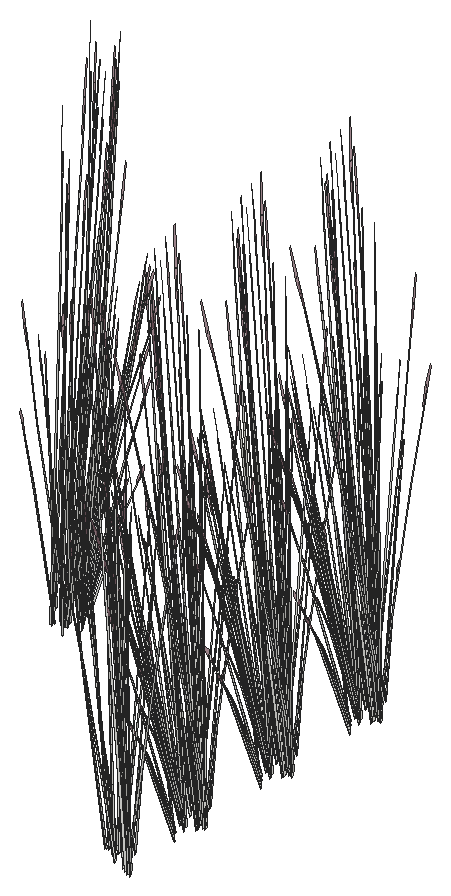
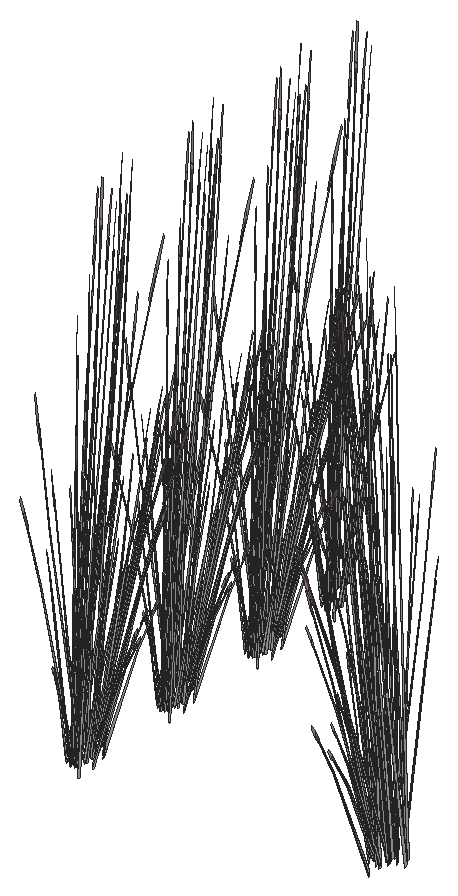
# SketchUp Ruby script. Lengths in inches.
U = 1.inch
M = Sketchup.active_model
def pt(a) = Geom::Point3d.new(a.map { |v| v * U })
def face(e, loops, mat)
  f = e.add_face(loops[0].map { |a| pt(a) })
  loops[1..].each { |l| e.add_face(l.map { |a| pt(a) }).erase! }
  f.material = f.back_material = mat if mat
  f
end
# faces: each face lists its corners as indices into pts; further lists are holes
def faces(e, pts, list, mat = nil) = list.each { |f| face(e, (f[0].is_a?(Array) ? f : [f]).map { |l| l.map { |i| pts[i] } }, mat) }
# xy, xz, yz: faces in a plane at the given z, y or x. An outline is a flat list of corners, or four numbers for a rectangle; further outlines are holes
def ring(l) = l.size == 4 ? [[l[0], l[1]], [l[2], l[1]], [l[2], l[3]], [l[0], l[3]]] : l.each_slice(2).to_a
def flat(e, list, mat, &to3) = list.each { |f| face(e, (f[0].is_a?(Array) ? f : [f]).map { |l| ring(l).map { |u, v| to3.(u, v) } }, mat) }
def xy(e, z, list, mat = nil) = flat(e, list, mat) { |x, y| [x, y, z] }
def xz(e, y, list, mat = nil) = flat(e, list, mat) { |x, z| [x, y, z] }
def yz(e, x, list, mat = nil) = flat(e, list, mat) { |y, z| [x, y, z] }
def lines(e, pts, list) = list.each { |a, b| e.add_line(pt(pts[a]), pt(pts[b])) }
# prism: a flat outline (further loops are holes) pulled along v
def prism(e, loops, v, mat = nil)
  f = face(e, loops, mat); d = Geom::Vector3d.new(v.map { |x| x * U })
  f.pushpull(f.normal.samedirection?(d) ? d.length : -d.length)
end
def box(e, o, s, mat = nil) = prism(e, [[o, [o[0] + s[0], o[1], o[2]], [o[0] + s[0], o[1] + s[1], o[2]], [o[0], o[1] + s[1], o[2]]]], [0, 0, s[2]], mat)
def at(x, y, z, deg = 0) = Geom::Transformation.translation(pt([x, y, z])) * Geom::Transformation.rotation(ORIGIN, Z_AXIS, deg.degrees)
def axes(o, x, y, z) = Geom::Transformation.new([*x, 0, *y, 0, *z, 0, *pt(o).to_a, 1])
def part(name) = M.definitions.add(name)
# library, detail: a bought-in or finely detailed component or shape, given as its bounding box
def library(name, o, s) = part(name).tap { |d| box(d.entities, o, s) }
def detail(e, o, s) = box(e.add_group.entities, o, s)
def put(e, d, t, mat = nil) = e.add_instance(d, t).tap { |i| i.material = mat if mat }
def group(e, t, mat = nil) = e.add_group.tap { |g| g.transformation = t; g.material = mat if mat }.entities
root = M.entities
M.materials.add("LightPink_Translucent").color = [144, 107, 117]
M.materials["LightPink_Translucent"].alpha = 0.75
c1 = part("blade")
p = [[2.15,0.21,22],[0,0.17,0],[0.09,0.45,0],[2.18,0.31,22],[2.29,0.31,22],[0.38,0.45,0],
  [2.48,0.24,33],[2.49,0.24,33],[2.48,0.22,33]]
faces(c1.entities,p,[[0,1,2,3],[4,5,2,3],[6,3,4,7],[8,0,3,6]])
c2 = part("seeds")
p = [[0.3,-0.1,1.38],[-0.01,-0.03,1.59],[-0.01,-0.03,0.03],[0.14,-0.07,-0.07],[0.29,-0.03,3],[0.15,0.01,3.11]]
faces(c2.entities,p,[[0,1,2,3],[1,0,4,5]],"LightPink_Translucent")
c3 = part("blade with seeds")
put(c3.entities,c1,at(0,0,0))
put(c3.entities,c2,axes([2.4,0.25,30.99],[1.5799,-0.05474,1.17369],[-0.12525,1.92788,0.29478],[-0.07173,-0.02425,1.56792]))
put(root,c3,axes([400.33,754.45,4.53],[-0.29332,-0.1301,-0.35414],[0.08555,-0.37955,0.4572],[-0.11809,0.0348,0.87481]))
put(root,c3,axes([401.96,755.35,2.67],[-0.35635,0.30962,-0.29095],[-0.23697,-0.43749,-0.50002],[-0.08792,-0.04443,1.59708]))
put(root,c3,axes([401.93,755.49,2.62],[-0.06809,0.4162,0.1448],[-0.33266,-0.07225,-0.41347],[-0.06054,-0.04274,1.26744]))
put(root,c3,axes([401.22,754.38,3.34],[0.10032,-0.06746,1.77064],[0.0346,0.47103,0.13857],[-0.2173,0.0625,0.63284]))
put(root,c3,axes([402.36,755.49,2.46],[-0.34464,-0.37536,-0.25192],[0.29,-0.42149,0.5513],[-0.0928,0.04391,1.68216]))
put(root,c3,axes([401.45,756.21,2.48],[0.33032,0.23318,0.49651],[-0.19744,0.41812,0],[-0.07523,-0.05311,1.57504]))
put(root,c3,axes([400.53,754.64,4.68],[-0.09562,0.42421,-0.51099],[-0.32782,-0.1454,-0.3958],[-0.13199,0.0389,0.97773]))
put(root,c3,axes([401.26,756.46,2.375],[-0.22066,0.46731,0],[-0.36918,-0.26061,-0.51607],[-0.08408,-0.05936,1.63711]))
put(root,c3,axes([402.1875,755.41,2.21],[-0.38326,0.02879,-0.44739],[-0.03466,-0.47788,0.21531],[-0.06861,0.04843,1.43643]))
put(root,c3,axes([400.52,754.86,3.875],[0.12246,-0.09864,1.71376],[0.1031,0.45582,0.13857],[-0.19225,0.10302,0.73262]))
put(root,c3,axes([400.14,755.64,2.59],[0.12266,0.03828,1.43002],[0.07906,0.39104,-0.30754],[-0.16661,0.0732,0.61141]))
put(root,c3,axes([399.88,756.46,2.77],[0.14709,-0.21136,1.1486],[0.05804,0.3346,0.84392],[-0.1063,0.05991,0.25299]))
put(root,c3,axes([400.43,755.54,4.53],[-0.30722,0.06665,-0.35414],[-0.08112,-0.381,0.4572],[-0.08804,0.10234,0.87481]))
put(root,c3,axes([402.2,755.6875,2.06],[-0.23773,0.35053,-0.62353],[-0.29532,-0.31785,-0.16365],[-0.09526,0.08744,1.37633]))
put(root,c3,axes([400.97,755.17,3.875],[0.08815,-0.14329,1.71376],[0.22258,0.38678,0.13857],[-0.15267,0.17614,0.73262]))
put(root,c3,axes([400.6875,755.59,4.68],[0.09067,0.42583,-0.51099],[-0.34336,0.07449,-0.3958],[-0.0984,0.11438,0.97773]))
put(root,c3,axes([400.27,756.67,1.49],[0.04734,0.04659,1.76342],[0.08027,0.4317,-0.26939],[-0.10492,0.09206,0.30037]))
put(root,c3,axes([400.9,755.52,3.875],[0.06572,-0.16029,1.71376],[0.27569,0.33172,0.13857],[-0.12437,0.20675,0.73262]))
put(root,c3,axes([400.98,756.42,4.53],[-0.23881,0.24554,-0.35414],[-0.22606,-0.28036,0.4572],[-0.0344,0.14245,0.87481]))
put(root,c3,axes([401.13,757.38,2.77],[-0.00913,-0.2773,1.1486],[0.22824,0.19778,0.84392],[-0.04489,0.13217,0.25299]))
put(root,c3,axes([401.27,763.66,3.875],[0.08068,0.14973,1.71376],[-0.3728,0.12606,0.13857],[-0.08426,-0.23506,0.73262]))
put(root,c3,axes([401.17,763.26,2.59],[-0.02137,0.15256,1.43002],[-0.31245,0.12771,-0.30754],[-0.07303,-0.19719,0.61141]))
put(root,c3,axes([401.13,756.16,5.34],[-0.00918,0.43138,-0.7886],[-0.38672,-0.02897,0.09517],[-0.04081,0.18275,1.11556]))
put(root,c3,axes([400.86,757.13,2.59],[0.11138,-0.07357,1.43002],[0.27499,0.22183,-0.30754],[-0.08185,0.19194,0.61141]))
put(root,c3,axes([401.0625,763.01,2.77],[0.18411,0.16231,1.1486],[-0.26813,0.09757,0.84392],[-0.05737,-0.12474,0.25299]))
put(root,c3,axes([401.51,763.875,4.98],[-0.30095,-0.22541,-0.71045],[0.21388,-0.395,0.08574],[-0.10904,-0.13459,1.00501]))
put(root,c3,axes([401.4,763.58,4.53],[-0.05451,-0.37564,-0.35414],[0.31161,-0.09919,0.4572],[-0.0837,-0.10765,0.87481]))
put(root,c3,axes([401.01,756.77,3.36],[0.00775,-0.24075,1.54345],[0.34877,0.12716,0.21329],[-0.03022,0.25658,0.72882]))
put(root,c3,axes([400.92,763.5,1.49],[-0.03419,0.06144,1.76342],[-0.3455,0.13246,-0.26939],[-0.08346,-0.12049,0.30037]))
put(root,c3,axes([400.73,764.12,3.875],[0.1311,0.08035,1.71376],[-0.27131,0.33708,0.13857],[-0.16909,-0.15206,0.73262]))
put(root,c3,axes([401.37,763.89,4.68],[-0.34827,0.11086,-0.51099],[-0.06092,-0.41983,-0.3958],[-0.09354,-0.12031,0.97773]))
put(root,c3,axes([402.23,766.42,3.33],[0.305,0.18805,1.51261],[-0.29879,0.40513,0.59816],[-0.13384,-0.24012,1.26806]))
put(root,c3,axes([400.68,764.24,4.53],[-0.20082,-0.29199,-0.35414],[0.2293,-0.2764,0.4572],[-0.1165,-0.04206,0.87481]))
put(root,c3,axes([400.7,763.74,2.13],[-0.10181,0.3808,-0.03893],[-0.31336,-0.11714,-0.17649],[-0.04758,-0.06228,0.58215]))
put(root,c3,axes([400.53,765.48,2.375],[-0.44133,0,0],[0,-0.52122,-0.51607],[0,-0.11871,1.63711]))
put(root,c3,axes([400.61,764.55,2.59],[0.06891,0.12984,1.43002],[-0.15879,0.35293,-0.30754],[-0.16304,-0.08436,0.61141]))
put(root,c3,axes([400.89,764.43,4.98],[-0.35281,-0.01123,-0.71045],[0.0237,-0.47284,0.08574],[-0.14947,-0.0499,1.00501]))
put(root,c3,axes([400.875,765.34,2.33],[-0.32829,0.39208,0.30756],[-0.32849,-0.38796,-0.36492],[-0.01146,-0.11134,1.64885]))
put(root,c3,axes([401.77,766.16,2.4375],[0.09355,-0.55261,-0.23429],[0.44354,0.09633,0.51271],[-0.0775,-0.07631,1.5644]))
put(root,c3,axes([400.78,764.53,4.68],[-0.25628,0.30892,-0.51099],[-0.22444,-0.32634,-0.3958],[-0.13021,-0.047,0.97773]))
put(root,c3,axes([400.2,764.9375,2.77],[0.22533,-0.03337,1.1486],[-0.14293,0.29403,0.84392],[-0.11135,-0.04411,0.25299]))
put(root,c3,axes([400.46,764.86,3.875],[0.14639,-0.01056,1.71376],[-0.09712,0.45778,0.13857],[-0.20862,-0.02831,0.73262]))
put(root,c3,axes([401.73,765.93,2.21],[-0.21202,-0.39143,-0.44739],[0.32115,-0.27564,0.21531],[-0.06861,-0.04843,1.43643]))
put(root,c3,axes([401.54,766.08,2.06],[-0.36714,-0.07646,-0.62353],[0.07747,-0.47163,-0.16365],[-0.10956,-0.05715,1.37633]))
put(root,c3,axes([400.36,765.42,1.49],[0.00895,0.0735,1.76342],[-0.18044,0.38382,-0.26939],[-0.12817,-0.01935,0.30037]))
put(root,c3,axes([401.15,766.8,2.03],[-0.08291,-0.40636,-0.30978],[0.32928,-0.11539,0.30978],[-0.06638,-0.04686,1.38974]))
put(root,c3,axes([401.0625,766.98,2.02],[-0.33032,-0.23318,-0.49651],[0.19744,-0.41812,0],[-0.07523,-0.05311,1.57504]))
put(root,c3,axes([400.33,765.25,4.53],[-0.29332,-0.1301,-0.35414],[0.08555,-0.37955,0.4572],[-0.11809,0.0348,0.87481]))
put(root,c3,axes([401.96,766.15,2.67],[-0.35635,0.30962,-0.29095],[-0.23697,-0.43749,-0.50002],[-0.08792,-0.04443,1.59708]))
put(root,c3,axes([401.93,766.29,2.62],[-0.06809,0.4162,0.1448],[-0.33266,-0.07225,-0.41347],[-0.06054,-0.04274,1.26744]))
put(root,c3,axes([401.22,765.1875,3.34],[0.10032,-0.06746,1.77064],[0.0346,0.47103,0.13857],[-0.2173,0.0625,0.63284]))
put(root,c3,axes([402.36,766.29,2.46],[-0.34464,-0.37536,-0.25192],[0.29,-0.42149,0.5513],[-0.0928,0.04391,1.68216]))
put(root,c3,axes([401.45,767.01,2.48],[0.33032,0.23318,0.49651],[-0.19744,0.41812,0],[-0.07523,-0.05311,1.57504]))
put(root,c3,axes([400.53,765.44,4.68],[-0.09562,0.42421,-0.51099],[-0.32782,-0.1454,-0.3958],[-0.13199,0.0389,0.97773]))
put(root,c3,axes([401.26,767.26,2.375],[-0.22066,0.46731,0],[-0.36918,-0.26061,-0.51607],[-0.08408,-0.05936,1.63711]))
put(root,c3,axes([402.1875,766.22,2.21],[-0.38326,0.02879,-0.44739],[-0.03466,-0.47788,0.21531],[-0.06861,0.04843,1.43643]))
put(root,c3,axes([400.52,765.66,3.875],[0.12246,-0.09864,1.71376],[0.1031,0.45582,0.13857],[-0.19225,0.10302,0.73262]))
put(root,c3,axes([400.14,766.44,2.59],[0.12266,0.03828,1.43002],[0.07906,0.39104,-0.30754],[-0.16661,0.0732,0.61141]))
put(root,c3,axes([399.88,767.26,2.77],[0.14709,-0.21136,1.1486],[0.05804,0.3346,0.84392],[-0.1063,0.05991,0.25299]))
put(root,c3,axes([400.43,766.34,4.53],[-0.30722,0.06665,-0.35414],[-0.08112,-0.381,0.4572],[-0.08804,0.10234,0.87481]))
put(root,c3,axes([402.2,766.49,2.06],[-0.23773,0.35053,-0.62353],[-0.29532,-0.31785,-0.16365],[-0.09526,0.08744,1.37633]))
put(root,c3,axes([400.97,765.97,3.875],[0.08815,-0.14329,1.71376],[0.22258,0.38678,0.13857],[-0.15267,0.17614,0.73262]))
put(root,c3,axes([400.6875,766.39,4.68],[0.09067,0.42583,-0.51099],[-0.34336,0.07449,-0.3958],[-0.0984,0.11438,0.97773]))
put(root,c3,axes([400.27,767.48,1.49],[0.04734,0.04659,1.76342],[0.08027,0.4317,-0.26939],[-0.10492,0.09206,0.30037]))
put(root,c3,axes([400.9,766.32,3.875],[0.06572,-0.16029,1.71376],[0.27569,0.33172,0.13857],[-0.12437,0.20675,0.73262]))
put(root,c3,axes([400.98,767.23,4.53],[-0.23881,0.24554,-0.35414],[-0.22606,-0.28036,0.4572],[-0.0344,0.14245,0.87481]))
put(root,c3,axes([401.13,768.18,2.77],[-0.00913,-0.2773,1.1486],[0.22824,0.19778,0.84392],[-0.04489,0.13217,0.25299]))
put(root,c3,axes([401.13,766.97,5.34],[-0.00918,0.43138,-0.7886],[-0.38672,-0.02897,0.09517],[-0.04081,0.18275,1.11556]))
put(root,c3,axes([400.86,767.93,2.59],[0.11138,-0.07357,1.43002],[0.27499,0.22183,-0.30754],[-0.08185,0.19194,0.61141]))
put(root,c3,axes([401.01,767.58,3.36],[0.00775,-0.24075,1.54345],[0.34877,0.12716,0.21329],[-0.03022,0.25658,0.72882]))
put(root,c3,axes([401.27,776.03,3.875],[0.08068,0.14973,1.71376],[-0.3728,0.12606,0.13857],[-0.08426,-0.23506,0.73262]))
put(root,c3,axes([401.17,775.64,2.59],[-0.02137,0.15256,1.43002],[-0.31245,0.12771,-0.30754],[-0.07303,-0.19719,0.61141]))
put(root,c3,axes([401.0625,775.39,2.77],[0.18411,0.16231,1.1486],[-0.26813,0.09757,0.84392],[-0.05737,-0.12474,0.25299]))
put(root,c3,axes([401.51,776.25,4.98],[-0.30095,-0.22541,-0.71045],[0.21388,-0.395,0.08574],[-0.10904,-0.13459,1.00501]))
put(root,c3,axes([401.4,775.95,4.53],[-0.05451,-0.37564,-0.35414],[0.31161,-0.09919,0.4572],[-0.0837,-0.10765,0.87481]))
put(root,c3,axes([400.92,775.88,1.49],[-0.03419,0.06144,1.76342],[-0.3455,0.13246,-0.26939],[-0.08346,-0.12049,0.30037]))
put(root,c3,axes([400.73,776.5,3.875],[0.1311,0.08035,1.71376],[-0.27131,0.33708,0.13857],[-0.16909,-0.15206,0.73262]))
put(root,c3,axes([401.37,776.26,4.68],[-0.34827,0.11086,-0.51099],[-0.06092,-0.41983,-0.3958],[-0.09354,-0.12031,0.97773]))
put(root,c3,axes([402.23,778.8,3.33],[0.305,0.18805,1.51261],[-0.29879,0.40513,0.59816],[-0.13384,-0.24012,1.26806]))
put(root,c3,axes([400.68,776.61,4.53],[-0.20082,-0.29199,-0.35414],[0.2293,-0.2764,0.4572],[-0.1165,-0.04206,0.87481]))
put(root,c3,axes([400.7,776.12,2.13],[-0.10181,0.3808,-0.03893],[-0.31336,-0.11714,-0.17649],[-0.04758,-0.06228,0.58215]))
put(root,c3,axes([400.53,777.86,2.375],[-0.44133,0,0],[0,-0.52122,-0.51607],[0,-0.11871,1.63711]))
put(root,c3,axes([400.61,776.92,2.59],[0.06891,0.12984,1.43002],[-0.15879,0.35293,-0.30754],[-0.16304,-0.08436,0.61141]))
put(root,c3,axes([400.89,776.81,4.98],[-0.35281,-0.01123,-0.71045],[0.0237,-0.47284,0.08574],[-0.14947,-0.0499,1.00501]))
put(root,c3,axes([400.875,777.72,2.33],[-0.32829,0.39208,0.30756],[-0.32849,-0.38796,-0.36492],[-0.01146,-0.11134,1.64885]))
put(root,c3,axes([401.77,778.54,2.4375],[0.09355,-0.55261,-0.23429],[0.44354,0.09633,0.51271],[-0.0775,-0.07631,1.5644]))
put(root,c3,axes([400.78,776.9,4.68],[-0.25628,0.30892,-0.51099],[-0.22444,-0.32634,-0.3958],[-0.13021,-0.047,0.97773]))
put(root,c3,axes([400.2,777.3125,2.77],[0.22533,-0.03337,1.1486],[-0.14293,0.29403,0.84392],[-0.11135,-0.04411,0.25299]))
put(root,c3,axes([400.46,777.23,3.875],[0.14639,-0.01056,1.71376],[-0.09712,0.45778,0.13857],[-0.20862,-0.02831,0.73262]))
put(root,c3,axes([401.73,778.3125,2.21],[-0.21202,-0.39143,-0.44739],[0.32115,-0.27564,0.21531],[-0.06861,-0.04843,1.43643]))
put(root,c3,axes([401.54,778.46,2.06],[-0.36714,-0.07646,-0.62353],[0.07747,-0.47163,-0.16365],[-0.10956,-0.05715,1.37633]))
put(root,c3,axes([400.36,777.79,1.49],[0.00895,0.0735,1.76342],[-0.18044,0.38382,-0.26939],[-0.12817,-0.01935,0.30037]))
put(root,c3,axes([401.15,779.18,2.03],[-0.08291,-0.40636,-0.30978],[0.32928,-0.11539,0.30978],[-0.06638,-0.04686,1.38974]))
put(root,c3,axes([401.0625,779.35,2.02],[-0.33032,-0.23318,-0.49651],[0.19744,-0.41812,0],[-0.07523,-0.05311,1.57504]))
put(root,c3,axes([400.33,777.63,4.53],[-0.29332,-0.1301,-0.35414],[0.08555,-0.37955,0.4572],[-0.11809,0.0348,0.87481]))
put(root,c3,axes([401.96,778.53,2.67],[-0.35635,0.30962,-0.29095],[-0.23697,-0.43749,-0.50002],[-0.08792,-0.04443,1.59708]))
put(root,c3,axes([401.93,778.67,2.62],[-0.06809,0.4162,0.1448],[-0.33266,-0.07225,-0.41347],[-0.06054,-0.04274,1.26744]))
put(root,c3,axes([401.22,777.5625,3.34],[0.10032,-0.06746,1.77064],[0.0346,0.47103,0.13857],[-0.2173,0.0625,0.63284]))
put(root,c3,axes([402.36,778.67,2.46],[-0.34464,-0.37536,-0.25192],[0.29,-0.42149,0.5513],[-0.0928,0.04391,1.68216]))
put(root,c3,axes([401.45,779.39,2.48],[0.33032,0.23318,0.49651],[-0.19744,0.41812,0],[-0.07523,-0.05311,1.57504]))
put(root,c3,axes([400.53,777.82,4.68],[-0.09562,0.42421,-0.51099],[-0.32782,-0.1454,-0.3958],[-0.13199,0.0389,0.97773]))
put(root,c3,axes([401.26,779.63,2.375],[-0.22066,0.46731,0],[-0.36918,-0.26061,-0.51607],[-0.08408,-0.05936,1.63711]))
put(root,c3,axes([402.1875,778.59,2.21],[-0.38326,0.02879,-0.44739],[-0.03466,-0.47788,0.21531],[-0.06861,0.04843,1.43643]))
put(root,c3,axes([400.52,778.04,3.875],[0.12246,-0.09864,1.71376],[0.1031,0.45582,0.13857],[-0.19225,0.10302,0.73262]))
put(root,c3,axes([400.14,778.82,2.59],[0.12266,0.03828,1.43002],[0.07906,0.39104,-0.30754],[-0.16661,0.0732,0.61141]))
put(root,c3,axes([399.88,779.64,2.77],[0.14709,-0.21136,1.1486],[0.05804,0.3346,0.84392],[-0.1063,0.05991,0.25299]))
put(root,c3,axes([400.43,778.72,4.53],[-0.30722,0.06665,-0.35414],[-0.08112,-0.381,0.4572],[-0.08804,0.10234,0.87481]))
put(root,c3,axes([402.2,778.87,2.06],[-0.23773,0.35053,-0.62353],[-0.29532,-0.31785,-0.16365],[-0.09526,0.08744,1.37633]))
put(root,c3,axes([400.97,778.35,3.875],[0.08815,-0.14329,1.71376],[0.22258,0.38678,0.13857],[-0.15267,0.17614,0.73262]))
put(root,c3,axes([400.6875,778.77,4.68],[0.09067,0.42583,-0.51099],[-0.34336,0.07449,-0.3958],[-0.0984,0.11438,0.97773]))
put(root,c3,axes([400.27,779.85,1.49],[0.04734,0.04659,1.76342],[0.08027,0.4317,-0.26939],[-0.10492,0.09206,0.30037]))
put(root,c3,axes([400.9,778.7,3.875],[0.06572,-0.16029,1.71376],[0.27569,0.33172,0.13857],[-0.12437,0.20675,0.73262]))
put(root,c3,axes([400.98,779.6,4.53],[-0.23881,0.24554,-0.35414],[-0.22606,-0.28036,0.4572],[-0.0344,0.14245,0.87481]))
put(root,c3,axes([401.13,780.56,2.77],[-0.00913,-0.2773,1.1486],[0.22824,0.19778,0.84392],[-0.04489,0.13217,0.25299]))
put(root,c3,axes([368.77,786.53,2.59],[-0.10032,0.0944,1.43002],[-0.30046,-0.16522,-0.30754],[0.05569,-0.20547,0.61141]))
put(root,c3,axes([401.13,779.34,5.34],[-0.00918,0.43138,-0.7886],[-0.38672,-0.02897,0.09517],[-0.04081,0.18275,1.11556]))
put(root,c3,axes([369.01,787.23,4.98],[0.00918,-0.43138,-0.71045],[0.38672,0.02897,0.08574],[0.04081,-0.18275,1.00501]))
put(root,c3,axes([368.58,787.01,3.875],[-0.06572,0.16029,1.71376],[-0.27569,-0.33172,0.13857],[0.12437,-0.20675,0.73262]))
put(root,c3,axes([400.86,780.3125,2.59],[0.11138,-0.07357,1.43002],[0.27499,0.22183,-0.30754],[-0.08185,0.19194,0.61141]))
put(root,c3,axes([369.17,786.97,4.53],[0.23881,-0.24554,-0.35414],[0.22606,0.28036,0.4572],[0.0344,-0.14245,0.87481]))
put(root,c3,axes([401.01,779.95,3.36],[0.00775,-0.24075,1.54345],[0.34877,0.12716,0.21329],[-0.03022,0.25658,0.72882]))
put(root,c3,axes([369.47,786.82,1.49],[-0.05283,-0.03674,1.76342],[-0.13569,-0.41045,-0.26939],[0.09154,-0.11138,0.30037]))
put(root,c3,axes([401.27,788.8,3.875],[0.08068,0.14973,1.71376],[-0.3728,0.12606,0.13857],[-0.08426,-0.23506,0.73262]))
put(root,c3,axes([401.17,788.41,2.59],[-0.02137,0.15256,1.43002],[-0.31245,0.12771,-0.30754],[-0.07303,-0.19719,0.61141]))
put(root,c3,axes([369.47,787.98,4.98],[0.18436,-0.36797,-0.71045],[0.32306,0.26151,0.08574],[0.11008,-0.13332,1.00501]))
put(root,c3,axes([369.46,787.8,4.68],[-0.09067,-0.42583,-0.51099],[0.34336,-0.07449,-0.3958],[0.0984,-0.11438,0.97773]))
put(root,c3,axes([367.78,786.83,2.02],[0.33032,-0.23318,-0.49651],[0.19744,0.41812,0],[0.07523,-0.05311,1.57504]))
put(root,c3,axes([369.74,787.64,2.59],[-0.12609,-0.01381,1.43002],[-0.12917,-0.37055,-0.30754],[0.1549,-0.10482,0.61141]))
put(root,c3,axes([368.17,787.79,2.06],[0.23773,-0.35053,-0.62353],[0.29532,0.31785,-0.16365],[0.09526,-0.08744,1.37633]))
put(root,c3,axes([369.88,786.96,2.77],[-0.11756,0.2374,1.1486],[-0.10105,-0.31895,0.84392],[0.09709,-0.07992,0.25299]))
put(root,c3,axes([369.71,787.85,4.53],[0.30722,-0.06665,-0.35414],[0.08112,0.381,0.4572],[0.08804,-0.10234,0.87481]))
put(root,c3,axes([401.0625,788.16,2.77],[0.18411,0.16231,1.1486],[-0.26813,0.09757,0.84392],[-0.05737,-0.12474,0.25299]))
put(root,c3,axes([401.51,789.02,4.98],[-0.30095,-0.22541,-0.71045],[0.21388,-0.395,0.08574],[-0.10904,-0.13459,1.00501]))
put(root,c3,axes([401.4,788.72,4.53],[-0.05451,-0.37564,-0.35414],[0.31161,-0.09919,0.4572],[-0.0837,-0.10765,0.87481]))
put(root,c3,axes([367.85,787.02,2.03],[0.32928,0.11539,-0.30978],[-0.08291,0.40636,0.30978],[0.06638,-0.04686,1.38974]))
put(root,c3,axes([400.92,788.65,1.49],[-0.03419,0.06144,1.76342],[-0.3455,0.13246,-0.26939],[-0.08346,-0.12049,0.30037]))
put(root,c3,axes([400.73,789.27,3.875],[0.1311,0.08035,1.71376],[-0.27131,0.33708,0.13857],[-0.16909,-0.15206,0.73262]))
put(root,c3,axes([401.37,789.03,4.68],[-0.34827,0.11086,-0.51099],[-0.06092,-0.41983,-0.3958],[-0.09354,-0.12031,0.97773]))
put(root,c3,axes([369.62,788.75,4.68],[0.09562,-0.42421,-0.51099],[0.32782,0.1454,-0.3958],[0.13199,-0.0389,0.97773]))
put(root,c3,axes([369.1,787.02,2.375],[0.22066,-0.46731,0],[0.36918,0.26061,-0.51607],[0.08408,0.05936,1.63711]))
put(root,c3,axes([402.23,791.57,3.33],[0.305,0.18805,1.51261],[-0.29879,0.40513,0.59816],[-0.13384,-0.24012,1.26806]))
put(root,c3,axes([369.97,788.87,1.98],[-0.22732,0.05597,1.41583],[-0.03618,-0.44548,0.08104],[0.15921,-0.06743,0.80566]))
put(root,c3,axes([370.38,788.48,2.26],[-0.21881,-0.29821,-0.06488],[0.23965,-0.27324,-0.29416],[0.0679,-0.01924,0.97024]))
put(root,c3,axes([368.91,787.27,2.48],[-0.33032,-0.23318,0.49651],[0.19744,-0.41812,0],[0.07523,0.05311,1.57504]))
put(root,c3,axes([369.56,788.9,4.98],[0.31014,-0.20596,-0.71045],[0.17284,0.42397,0.08574],[0.14985,-0.04816,1.00501]))
put(root,c3,axes([400.68,789.38,4.53],[-0.20082,-0.29199,-0.35414],[0.2293,-0.2764,0.4572],[-0.1165,-0.04206,0.87481]))
put(root,c3,axes([367.51,787.85,1.59],[-0.3474,0.18671,1.28929],[-0.11057,-0.53572,0.50096],[0.21332,0.00891,1.46642]))
put(root,c3,axes([368.4375,787.99,2.62],[0.06809,-0.4162,0.1448],[0.33266,0.07225,-0.41347],[0.06054,0.04274,1.26744]))
put(root,c3,axes([370.22,788.58,1.49],[-0.01845,-0.0708,1.76342],[0.12793,-0.41416,-0.26939],[0.12905,-0.00596,0.30037]))
put(root,c3,axes([400.7,788.89,2.13],[-0.10181,0.3808,-0.03893],[-0.31336,-0.11714,-0.17649],[-0.04758,-0.06228,0.58215]))
put(root,c3,axes([400.53,790.625,2.375],[-0.44133,0,0],[0,-0.52122,-0.51607],[0,-0.11871,1.63711]))
put(root,c3,axes([400.61,789.69,2.59],[0.06891,0.12984,1.43002],[-0.15879,0.35293,-0.30754],[-0.16304,-0.08436,0.61141]))
put(root,c3,axes([400.89,789.58,4.98],[-0.35281,-0.01123,-0.71045],[0.0237,-0.47284,0.08574],[-0.14947,-0.0499,1.00501]))
put(root,c3,axes([368.41,788.13,2.67],[0.35635,-0.30962,-0.29095],[0.23697,0.43749,-0.50002],[0.08792,0.04443,1.59708]))
put(root,c3,axes([369.82,788.94,4.53],[0.29332,0.1301,-0.35414],[-0.08555,0.37955,0.4572],[0.11809,-0.0348,0.87481]))
put(root,c3,axes([369.3,787.3,2.02],[0.33032,0.23318,-0.49651],[-0.19744,0.41812,0],[0.07523,0.05311,1.57504]))
put(root,c3,axes([369.02,788.47,3.875],[-0.14639,0.01056,1.71376],[0.09712,-0.45778,0.13857],[0.20862,0.02831,0.73262]))
put(root,c3,axes([369.21,787.48,2.03],[0.08291,0.40636,-0.30978],[-0.32928,0.11539,0.30978],[0.06638,0.04686,1.38974]))
put(root,c3,axes([400.875,790.49,2.33],[-0.32829,0.39208,0.30756],[-0.32849,-0.38796,-0.36492],[-0.01146,-0.11134,1.64885]))
put(root,c3,axes([401.77,791.3,2.4375],[0.09355,-0.55261,-0.23429],[0.44354,0.09633,0.51271],[-0.0775,-0.07631,1.5644]))
put(root,c3,axes([400.78,789.67,4.68],[-0.25628,0.30892,-0.51099],[-0.22444,-0.32634,-0.3958],[-0.13021,-0.047,0.97773]))
put(root,c3,axes([368.625,789.7,2.18],[0.37054,-0.15823,-0.19198],[0.1302,0.45581,0.00008],[0.0409,-0.01749,1.73897]))
put(root,c3,axes([400.2,790.08,2.77],[0.22533,-0.03337,1.1486],[-0.14293,0.29403,0.84392],[-0.11135,-0.04411,0.25299]))
put(root,c3,axes([368.82,788.2,2.06],[0.36714,0.07646,-0.62353],[-0.07747,0.47163,-0.16365],[0.10956,0.05715,1.37633]))
put(root,c3,axes([370.44,789.02,2.77],[-0.21807,0.07699,1.1486],[0.10265,-0.31819,0.84392],[0.11568,0.02177,0.25299]))
put(root,c3,axes([400.46,790,3.875],[0.14639,-0.01056,1.71376],[-0.09712,0.45778,0.13857],[-0.20862,-0.02831,0.73262]))
put(root,c3,axes([401.73,791.08,2.21],[-0.21202,-0.39143,-0.44739],[0.32115,-0.27564,0.21531],[-0.06861,-0.04843,1.43643]))
put(root,c3,axes([368.63,788.35,2.21],[0.21202,0.39143,-0.44739],[-0.32115,0.27564,0.21531],[0.06861,0.04843,1.43643]))
put(root,c3,axes([370.06,790,3.93],[-0.06755,-0.39203,-0.03492],[0.31928,-0.09013,-0.15832],[0.06667,0.02485,0.52218]))
put(root,c3,axes([369.5625,788.72,2.48],[0,-0.46636,0.49651],[0.39487,0,0],[0,0.10622,1.57504]))
put(root,c3,axes([401.54,791.23,2.06],[-0.36714,-0.07646,-0.62353],[0.07747,-0.47163,-0.16365],[-0.10956,-0.05715,1.37633]))
put(root,c3,axes([370.03,789.53,2.59],[-0.085,-0.1147,1.43002],[0.1106,-0.37943,-0.30754],[0.17198,0.0514,0.61141]))
put(root,c3,axes([400.36,790.5625,1.49],[0.00895,0.0735,1.76342],[-0.18044,0.38382,-0.26939],[-0.12817,-0.01935,0.30037]))
put(root,c3,axes([401.15,791.95,2.03],[-0.08291,-0.40636,-0.30978],[0.32928,-0.11539,0.30978],[-0.06638,-0.04686,1.38974]))
put(root,c3,axes([401.0625,792.12,2.02],[-0.33032,-0.23318,-0.49651],[0.19744,-0.41812,0],[-0.07523,-0.05311,1.57504]))
put(root,c3,axes([400.33,790.4,4.53],[-0.29332,-0.1301,-0.35414],[0.08555,-0.37955,0.4572],[-0.11809,0.0348,0.87481]))
put(root,c3,axes([369.25,789.76,4.98],[0.35281,0.01123,-0.71045],[-0.0237,0.47284,0.08574],[0.14947,0.0499,1.00501]))
put(root,c3,axes([401.96,791.3,2.67],[-0.35635,0.30962,-0.29095],[-0.23697,-0.43749,-0.50002],[-0.08792,-0.04443,1.59708]))
put(root,c3,axes([369.83,788.8,2.375],[0.44133,0,0],[0,0.52122,-0.51607],[0,0.11871,1.63711]))
put(root,c3,axes([368.7,788.62,2.67],[0.39748,0.22252,-0.29095],[-0.19139,0.46966,-0.50002],[0.01249,0.11531,1.59708]))
put(root,c3,axes([369.47,789.96,4.53],[0.20082,0.29199,-0.35414],[-0.2293,0.2764,0.4572],[0.1165,0.04206,0.87481]))
put(root,c3,axes([401.93,791.43,2.62],[-0.06809,0.4162,0.1448],[-0.33266,-0.07225,-0.41347],[-0.06054,-0.04274,1.26744]))
put(root,c3,axes([401.22,790.33,3.34],[0.10032,-0.06746,1.77064],[0.0346,0.47103,0.13857],[-0.2173,0.0625,0.63284]))
put(root,c3,axes([402.36,791.44,2.46],[-0.34464,-0.37536,-0.25192],[0.29,-0.42149,0.5513],[-0.0928,0.04391,1.68216]))
put(root,c3,axes([401.45,792.16,2.48],[0.33032,0.23318,0.49651],[-0.19744,0.41812,0],[-0.07523,-0.05311,1.57504]))
put(root,c3,axes([369.73,789.16,2.02],[0,0.46636,-0.49651],[-0.39487,0,0],[0,0.10622,1.57504]))
put(root,c3,axes([368.75,789.21,3.875],[-0.1311,-0.08035,1.71376],[0.27131,-0.33708,0.13857],[0.16909,0.15206,0.73262]))
put(root,c3,axes([400.53,790.59,4.68],[-0.09562,0.42421,-0.51099],[-0.32782,-0.1454,-0.3958],[-0.13199,0.0389,0.97773]))
put(root,c3,axes([401.26,792.4,2.375],[-0.22066,0.46731,0],[-0.36918,-0.26061,-0.51607],[-0.08408,-0.05936,1.63711]))
put(root,c3,axes([369.23,790.125,2.77],[-0.19872,-0.13409,1.1486],[0.2566,-0.13625,0.84392],[0.06921,0.11541,0.25299]))
put(root,c3,axes([402.1875,791.36,2.21],[-0.38326,0.02879,-0.44739],[-0.03466,-0.47788,0.21531],[-0.06861,0.04843,1.43643]))
put(root,c3,axes([369.29,790.62,1.49],[0.02571,-0.06733,1.76342],[0.32373,-0.19829,-0.26939],[0.09815,0.10263,0.30037]))
put(root,c3,axes([368.78,790.31,4.68],[0.34827,-0.11086,-0.51099],[0.06092,0.41983,-0.3958],[0.09354,0.12031,0.97773]))
put(root,c3,axes([400.52,790.81,3.875],[0.12246,-0.09864,1.71376],[0.1031,0.45582,0.13857],[-0.19225,0.10302,0.73262]))
put(root,c3,axes([369.26,790.73,2.67],[-0.22633,-0.01463,1.0506],[0.14947,-0.31064,0.58006],[0.08941,0.11036,0.8241]))
put(root,c3,axes([400.14,791.59,2.59],[0.12266,0.03828,1.43002],[0.07906,0.39104,-0.30754],[-0.16661,0.0732,0.61141]))
put(root,c3,axes([368.52,789.98,2.59],[0.00623,-0.15459,1.43002],[0.29764,-0.17268,-0.30754],[0.09188,0.18503,0.61141]))
put(root,c3,axes([399.88,792.4,2.77],[0.14709,-0.21136,1.1486],[0.05804,0.3346,0.84392],[-0.1063,0.05991,0.25299]))
put(root,c3,axes([400.43,791.49,4.53],[-0.30722,0.06665,-0.35414],[-0.08112,-0.381,0.4572],[-0.08804,0.10234,0.87481]))
put(root,c3,axes([402.2,791.64,2.06],[-0.23773,0.35053,-0.62353],[-0.29532,-0.31785,-0.16365],[-0.09526,0.08744,1.37633]))
put(root,c3,axes([368.21,789.68,3.875],[-0.08068,-0.14973,1.71376],[0.3728,-0.12606,0.13857],[0.08426,0.23506,0.73262]))
put(root,c3,axes([400.97,791.12,3.875],[0.08815,-0.14329,1.71376],[0.22258,0.38678,0.13857],[-0.15267,0.17614,0.73262]))
put(root,c3,axes([400.6875,791.54,4.68],[0.09067,0.42583,-0.51099],[-0.34336,0.07449,-0.3958],[-0.0984,0.11438,0.97773]))
put(root,c3,axes([400.27,792.62,1.49],[0.04734,0.04659,1.76342],[0.08027,0.4317,-0.26939],[-0.10492,0.09206,0.30037]))
put(root,c3,axes([400.9,791.47,3.875],[0.06572,-0.16029,1.71376],[0.27569,0.33172,0.13857],[-0.12437,0.20675,0.73262]))
put(root,c3,axes([400.98,792.37,4.53],[-0.23881,0.24554,-0.35414],[-0.22606,-0.28036,0.4572],[-0.0344,0.14245,0.87481]))
put(root,c3,axes([401.13,793.33,2.77],[-0.00913,-0.2773,1.1486],[0.22824,0.19778,0.84392],[-0.04489,0.13217,0.25299]))
put(root,c3,axes([401.13,792.11,5.34],[-0.00918,0.43138,-0.7886],[-0.38672,-0.02897,0.09517],[-0.04081,0.18275,1.11556]))
put(root,c3,axes([400.86,793.08,2.59],[0.11138,-0.07357,1.43002],[0.27499,0.22183,-0.30754],[-0.08185,0.19194,0.61141]))
put(root,c3,axes([401.01,792.72,3.36],[0.00775,-0.24075,1.54345],[0.34877,0.12716,0.21329],[-0.03022,0.25658,0.72882]))
